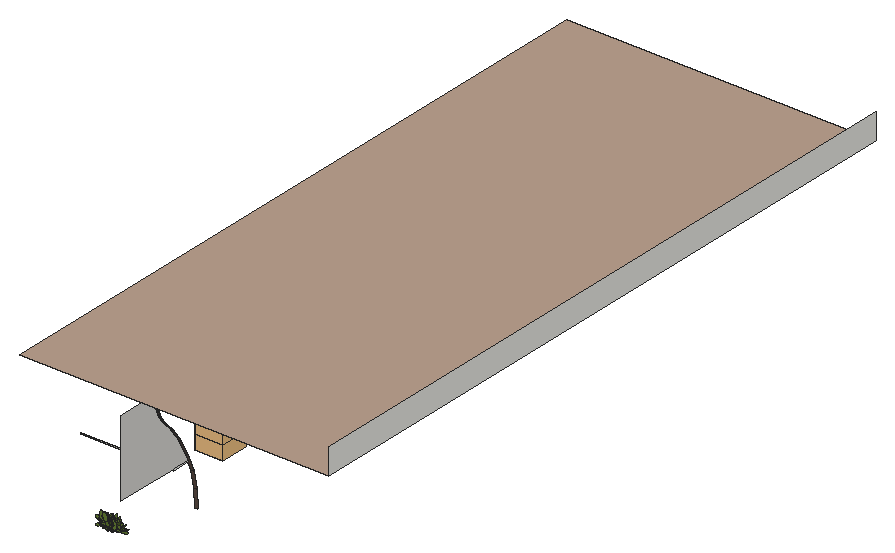
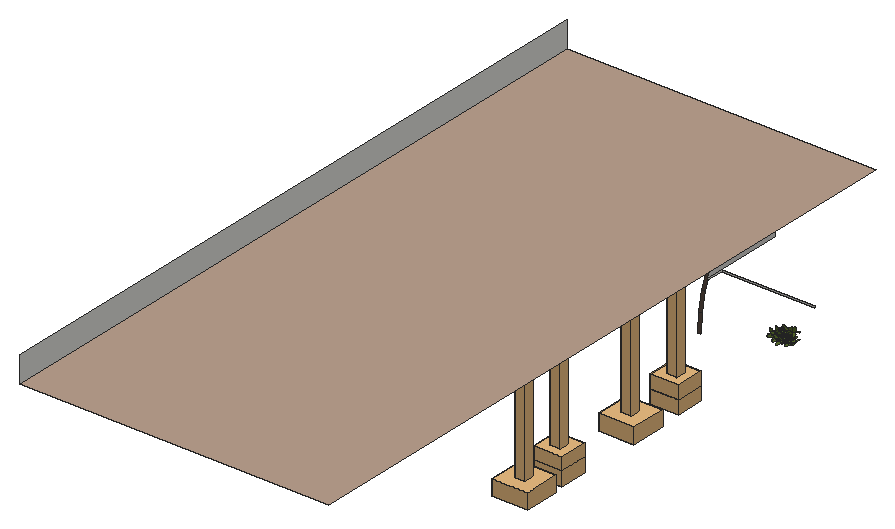
# SketchUp Ruby script. Lengths in inches.
U = 1.inch
M = Sketchup.active_model
def pt(a) = Geom::Point3d.new(a.map { |v| v * U })
def face(e, loops, mat)
  f = e.add_face(loops[0].map { |a| pt(a) })
  loops[1..].each { |l| e.add_face(l.map { |a| pt(a) }).erase! }
  f.material = f.back_material = mat if mat
  f
end
# faces: each face lists its corners as indices into pts; further lists are holes
def faces(e, pts, list, mat = nil) = list.each { |f| face(e, (f[0].is_a?(Array) ? f : [f]).map { |l| l.map { |i| pts[i] } }, mat) }
# xy, xz, yz: faces in a plane at the given z, y or x. An outline is a flat list of corners, or four numbers for a rectangle; further outlines are holes
def ring(l) = l.size == 4 ? [[l[0], l[1]], [l[2], l[1]], [l[2], l[3]], [l[0], l[3]]] : l.each_slice(2).to_a
def flat(e, list, mat, &to3) = list.each { |f| face(e, (f[0].is_a?(Array) ? f : [f]).map { |l| ring(l).map { |u, v| to3.(u, v) } }, mat) }
def xy(e, z, list, mat = nil) = flat(e, list, mat) { |x, y| [x, y, z] }
def xz(e, y, list, mat = nil) = flat(e, list, mat) { |x, z| [x, y, z] }
def yz(e, x, list, mat = nil) = flat(e, list, mat) { |y, z| [x, y, z] }
def lines(e, pts, list) = list.each { |a, b| e.add_line(pt(pts[a]), pt(pts[b])) }
# prism: a flat outline (further loops are holes) pulled along v
def prism(e, loops, v, mat = nil)
  f = face(e, loops, mat); d = Geom::Vector3d.new(v.map { |x| x * U })
  f.pushpull(f.normal.samedirection?(d) ? d.length : -d.length)
end
def box(e, o, s, mat = nil) = prism(e, [[o, [o[0] + s[0], o[1], o[2]], [o[0] + s[0], o[1] + s[1], o[2]], [o[0], o[1] + s[1], o[2]]]], [0, 0, s[2]], mat)
def at(x, y, z, deg = 0) = Geom::Transformation.translation(pt([x, y, z])) * Geom::Transformation.rotation(ORIGIN, Z_AXIS, deg.degrees)
def axes(o, x, y, z) = Geom::Transformation.new([*x, 0, *y, 0, *z, 0, *pt(o).to_a, 1])
def part(name) = M.definitions.add(name)
# library, detail: a bought-in or finely detailed component or shape, given as its bounding box
def library(name, o, s) = part(name).tap { |d| box(d.entities, o, s) }
def detail(e, o, s) = box(e.add_group.entities, o, s)
def put(e, d, t, mat = nil) = e.add_instance(d, t).tap { |i| i.material = mat if mat }
def group(e, t, mat = nil) = e.add_group.tap { |g| g.transformation = t; g.material = mat if mat }.entities
root = M.entities
M.materials.add("2").color = [91, 76, 69]
M.materials.add("[0008_LavenderBlush]").color = [212, 210, 207]
M.materials.add("[Asphalt_New]").color = [85, 106, 44]
M.materials.add("[Color A01]4").color = [188, 161, 143]
M.materials.add("white").color = [255, 255, 255]
c1 = part("Component\#59")
xy(c1.entities,0,[[5.79,0,4.75,0.06,3.73,0.22,2.73,0.5,1.77,0.88,0.86,1.37,0,1.95,0.83,2.59,1.74,3.13,2.7,3.56,3.7,3.87,4.74,4.05,5.79,4.12,6.84,4.05,7.87,3.87,8.88,3.56,9.84,3.13,10.74,2.59,11.57,1.95,10.72,1.37,9.8,0.88,8.84,0.5,7.84,0.22,6.82,0.06]],"[Asphalt_New]")
c2 = part("Leaf cluster")
put(c2.entities,c1,axes([10.37,9.23,1.73],[-0.67725,-0.67301,0.29729],[0.61625,-0.73963,-0.27052],[0.40195,0,0.91566]),"[Asphalt_New]")
put(c2.entities,c1,at(0,5.84,1.2),"[Asphalt_New]")
put(c2.entities,c1,axes([11.625,9.72,1.52],[-0.61694,-0.11161,0.77906],[-0.02647,-0.98639,-0.16227],[0.78657,-0.12073,0.60559]),"[Asphalt_New]")
put(c2.entities,c1,axes([13.35,8.05,1.98],[-0.1211,0.99122,-0.05316],[-0.90762,-0.13226,-0.39842],[-0.40195,0,0.91566]),"[Asphalt_New]")
c3 = library("Pendant light \#1",[-0.17,-0.17,-2.13],[2.36,2.36,31.14])
c4 = library("Group\#191",[0,0,0],[4.97,5,2.25])
c5 = library("Pendant light",[-0.17,-0.17,-2.23],[2.36,2.36,33.73])
c6 = library("Group\#195",[0,0,0],[6.25,6.23,2.75])
xy(root,126,[[125.375,9,197.1875,167.625]],"[Color A01]4")
xz(root,24.3,[[127.1875,103.38,148.875,103.78]],"[0008_LavenderBlush]")
yz(root,148.875,[[24.3,103.38,24.3,103.78,28.3,103.78,28.45,103.38]])
yz(root,148.875,[[9,103.78,9,121.625,18.35,121.625,18.35,122.4375,18.37,121.69,18.43,120.95,18.53,120.22,18.6875,119.49,18.89,118.78,19.14,118.08,19.4375,117.39,19.77,116.73,20.16,116.09,20.58,115.48,21.04,114.9,21.54,114.35,23.03,112.8,25.57,109.32,27.63,105.54,28.3,103.78]],"[0008_LavenderBlush]")
yz(root,197.1875,[[9,126,167.625,132]])
p = [[148.875,30.14,97.33],[149.5625,30.14,97.33],[149.5625,30.54,93.04],[148.875,30.54,93.04],[148.875,29.16,101.52],[149.5625,29.16,101.52],
  [148.875,27.63,105.54],[149.5625,27.63,105.54],[148.875,28.45,103.38],[148.875,28.3,103.78],[148.875,25.57,109.32],[149.5625,25.57,109.32],
  [148.875,23.03,112.8],[149.5625,23.03,112.8],[148.875,21.54,114.35],[149.5625,21.54,114.35],[148.875,21.04,114.9],[149.5625,21.04,114.9],
  [148.875,20.58,115.48],[149.5625,20.58,115.48],[148.875,20.16,116.09],[149.5625,20.16,116.09],[148.875,19.77,116.73],[149.5625,19.77,116.73],
  [148.875,19.4375,117.39],[149.5625,19.4375,117.39],[148.875,19.14,118.08],[149.5625,19.14,118.08],[148.875,18.89,118.78],[149.5625,18.89,118.78],
  [148.875,18.6875,119.49],[149.5625,18.6875,119.49],[148.875,18.53,120.22],[149.5625,18.53,120.22],[148.875,18.43,120.95],[149.5625,18.43,120.95],
  [148.875,18.37,121.69],[149.5625,18.37,121.69],[148.875,20.04,115.9],[149.5625,20.04,115.9]]
faces(root,p,[[0,1,2,3],[4,5,1,0],[6,7,5,4,8,9],[10,11,7,6],[12,13,11,10],[14,15,13,12],[14,16,17,15],[16,18,19,17],
  [18,20,21,19],[20,22,23,21],[22,24,25,23],[24,26,27,25],[26,28,29,27],[28,30,31,29],[30,32,33,31],[32,34,35,33],
  [34,36,37,35]],"2")
lines(root,p,[[38,39]])
detail(root,[134.31,48.47,92.11],[6.61,6.57,3.23])
detail(root,[134.31,82.33,92.11],[6.61,6.58,3.23])
put(root,c2,axes([138.4,18.32,90.67],[0.09591,-0.11801,0],[0.11801,0.09591,0],[0,0,0.17792]),"white")
put(root,c1,axes([136.48,18.12,90.71],[0.15184,-0.00221,-0.00946],[-0.00119,0.13948,-0.07089],[0.0083,0.06056,0.16292]),"[Asphalt_New]")
put(root,c2,axes([139,20.15,91.62],[-0.12334,-0.08896,0],[0.08896,-0.12334,0],[0,0,0.17792]),"white")
put(root,c2,axes([135.4,18.39,91.69],[0.09591,-0.11801,0],[0.11801,0.09591,0],[0,0,0.17792]),"white")
put(root,c1,axes([140.22,17.88,90.63],[-0.00707,0.09508,0.13861],[-0.14876,0.01968,-0.02887],[-0.03076,-0.11704,0.10775]),"[Asphalt_New]")
put(root,c2,axes([139.48,16.79,90.46],[0.12739,0.08305,0],[-0.08305,0.12739,0],[0,0,0.17792]),"white")
put(root,c2,axes([137.25,16.8125,90.89],[0.12739,0.08305,0],[-0.08305,0.12739,0],[0,0,0.17792]),"white")
put(root,c2,axes([139.18,20.1875,90.75],[-0.10525,-0.10976,0],[0.10976,-0.10525,0],[0,0,0.17792]),"white")
put(root,c2,axes([139.1,19.04,90.54],[-0.12303,0.08939,0],[-0.08939,-0.12303,0],[0,0,0.17792]),"white")
put(root,c1,axes([137.73,19.46,90.58],[-0.02064,-0.15066,0],[0.15066,-0.02064,0],[0,0,0.17792]),"[Asphalt_New]")
put(root,c1,axes([137.57,17.66,90.93],[0.01807,0.15078,-0.00946],[-0.13884,0.01339,-0.07089],[-0.05936,0.01458,0.16292]),"[Asphalt_New]")
put(root,c1,axes([140.16,18.08,90.67],[-0.09102,0.11312,0.0529],[-0.12166,-0.08144,-0.04813],[-0.00639,-0.06079,0.16292]),"[Asphalt_New]")
put(root,c1,axes([138.08,18.27,90.71],[0.15183,0.00256,-0.00946],[-0.00557,0.13937,-0.07089],[0.00639,0.06079,0.16292]),"[Asphalt_New]")
put(root,c1,axes([140.07,17.97,90.42],[-0.00408,0.09525,0.13861],[-0.14807,0.02435,-0.02887],[-0.03442,-0.11602,0.10775]),"[Asphalt_New]")
put(root,c1,axes([140.79,17.75,90.67],[0.10299,0.10235,0.0529],[-0.09371,0.11248,-0.04813],[-0.06112,0,0.16292]),"[Asphalt_New]")
put(root,c2,axes([141.9,19.1,90.54],[-0.12303,0.08939,0],[-0.08939,-0.12303,0],[0,0,0.17792]),"white")
put(root,c2,axes([137.49,16.9,90.67],[0.12994,0.079,0],[-0.079,0.12994,0],[0,0,0.17792]),"white")
put(root,c1,axes([140.16,18.92,90.89],[-0.15207,0,0],[0,-0.15207,0],[0,0,0.17792]),"[Asphalt_New]")
put(root,c2,axes([136.17,18.03,91.48],[0.1271,-0.08349,0],[0.08349,0.1271,0],[0,0,0.17792]),"white")
put(root,c1,axes([137.79,17.82,91.69],[0.10299,0.10235,0.0529],[-0.09371,0.11248,-0.04813],[-0.06112,0,0.16292]),"[Asphalt_New]")
put(root,c1,axes([137.83,18.0625,90.85],[-0.00408,0.09525,0.13861],[-0.14807,0.02435,-0.02887],[-0.03442,-0.11602,0.10775]),"[Asphalt_New]")
put(root,c1,axes([140.02,18.17,90.46],[-0.08742,0.11593,0.0529],[-0.12415,-0.07758,-0.04813],[-0.0083,-0.06056,0.16292]),"[Asphalt_New]")
put(root,c1,axes([139.58,18.13,90.63],[-0.00707,0.09508,0.13861],[-0.14876,0.01968,-0.02887],[-0.03076,-0.11704,0.10775]),"[Asphalt_New]")
put(root,c1,axes([138.39,18.33,90.94],[0.09382,0.01697,0.13861],[0.00402,0.15,-0.02887],[-0.11961,0.01836,0.10775]),"[Asphalt_New]")
put(root,c1,axes([138.96,17.85,90.93],[0.01807,0.15078,-0.00946],[-0.13884,0.01339,-0.07089],[-0.05936,0.01458,0.16292]),"[Asphalt_New]")
put(root,c1,axes([137.79,18.26,90.88],[-0.08742,0.11593,0.0529],[-0.12415,-0.07758,-0.04813],[-0.0083,-0.06056,0.16292]),"[Asphalt_New]")
put(root,c2,axes([138.18,20.46,90.54],[-0.10525,-0.10976,0],[0.10976,-0.10525,0],[0,0,0.17792]),"white")
put(root,c1,axes([139.81,19.7,90.58],[-0.0159,-0.15124,0],[0.15124,-0.0159,0],[0,0,0.17792]),"[Asphalt_New]")
put(root,c2,axes([138.97,17.11,90.67],[0.12739,0.08305,0],[-0.08305,0.12739,0],[0,0,0.17792]),"white")
put(root,c1,axes([139.52,18.33,90.67],[-0.09102,0.11312,0.0529],[-0.12166,-0.08144,-0.04813],[-0.00639,-0.06079,0.16292]),"[Asphalt_New]")
put(root,c2,axes([136.53,20.4,90.52],[-0.06975,-0.13513,0],[0.13513,-0.06975,0],[0,0,0.17792]),"white")
put(root,c1,axes([139.73,19.8,90.36],[-0.02064,-0.15066,0],[0.15066,-0.02064,0],[0,0,0.17792]),"[Asphalt_New]")
put(root,c1,axes([139.5625,18.31,90.63],[-0.00408,0.09525,0.13861],[-0.14807,0.02435,-0.02887],[-0.03442,-0.11602,0.10775]),"[Asphalt_New]")
put(root,c1,axes([136.98,18.1,90.7],[-0.0255,0.1497,-0.00946],[-0.13692,-0.02659,-0.07089],[-0.06106,-0.00288,0.16292]),"[Asphalt_New]")
put(root,c1,axes([139.61,19.24,90.89],[-0.15207,0,0],[0,-0.15207,0],[0,0,0.17792]),"[Asphalt_New]")
put(root,c1,axes([140.07,18.67,90.5],[0.15183,0.00256,-0.00946],[-0.00557,0.13937,-0.07089],[0.00639,0.06079,0.16292]),"[Asphalt_New]")
put(root,c1,axes([137.49,19.89,90.79],[-0.02064,-0.15066,0],[0.15066,-0.02064,0],[0,0,0.17792]),"[Asphalt_New]")
put(root,c1,axes([137.83,18.7,90.93],[0.15183,0.00256,-0.00946],[-0.00557,0.13937,-0.07089],[0.00639,0.06079,0.16292]),"[Asphalt_New]")
put(root,c1,axes([139.52,18.51,90.67],[-0.08742,0.11593,0.0529],[-0.12415,-0.07758,-0.04813],[-0.0083,-0.06056,0.16292]),"[Asphalt_New]")
put(root,c1,axes([137.96,18.125,90.71],[0.01807,0.15078,-0.00946],[-0.13884,0.01339,-0.07089],[-0.05936,0.01458,0.16292]),"[Asphalt_New]")
put(root,c2,axes([136.19,18.96,90.98],[0.09591,-0.11801,0],[0.11801,0.09591,0],[0,0,0.17792]),"white")
put(root,c1,axes([138.14,18.77,90.71],[0.15184,-0.00221,-0.00946],[-0.00119,0.13948,-0.07089],[0.0083,0.06056,0.16292]),"[Asphalt_New]")
put(root,c1,axes([139.17,19.95,90.58],[-0.0159,-0.15124,0],[0.15124,-0.0159,0],[0,0,0.17792]),"[Asphalt_New]")
put(root,c1,axes([142.5,19.36,90.36],[-0.15207,0,0],[0,-0.15207,0],[0,0,0.17792]),"[Asphalt_New]")
put(root,c1,axes([137.84,18.65,90.94],[0.09382,0.01697,0.13861],[0.00402,0.15,-0.02887],[-0.11961,0.01836,0.10775]),"[Asphalt_New]")
put(root,c1,axes([138.36,18.5,90.63],[-0.00707,0.09508,0.13861],[-0.14876,0.01968,-0.02887],[-0.03076,-0.11704,0.10775]),"[Asphalt_New]")
put(root,c1,axes([140.73,18.78,90.42],[0.09382,0.01697,0.13861],[0.00402,0.15,-0.02887],[-0.11961,0.01836,0.10775]),"[Asphalt_New]")
put(root,c1,axes([138.3125,18.7,90.67],[-0.09102,0.11312,0.0529],[-0.12166,-0.08144,-0.04813],[-0.00639,-0.06079,0.16292]),"[Asphalt_New]")
put(root,c1,axes([138.58,18.4,90.98],[0.10299,0.10235,0.0529],[-0.09371,0.11248,-0.04813],[-0.06112,0,0.16292]),"[Asphalt_New]")
put(root,c1,axes([139.22,20.14,90.58],[-0.02064,-0.15066,0],[0.15066,-0.02064,0],[0,0,0.17792]),"[Asphalt_New]")
put(root,c2,axes([140.73,19.74,90.54],[-0.12303,0.08939,0],[-0.08939,-0.12303,0],[0,0,0.17792]),"white")
put(root,c1,axes([136.76,18.9375,90.71],[0.15183,0.00256,-0.00946],[-0.00557,0.13937,-0.07089],[0.00639,0.06079,0.16292]),"[Asphalt_New]")
put(root,c1,axes([136.42,20.17,90.58],[-0.02064,-0.15066,0],[0.15066,-0.02064,0],[0,0,0.17792]),"[Asphalt_New]")
put(root,c1,axes([139.55,19,90.71],[0.15183,0.00256,-0.00946],[-0.00557,0.13937,-0.07089],[0.00639,0.06079,0.16292]),"[Asphalt_New]")
put(root,c2,axes([135.65,19.29,90.98],[0.09591,-0.11801,0],[0.11801,0.09591,0],[0,0,0.17792]),"white")
put(root,c1,axes([137.96,20.32,90.58],[-0.0159,-0.15124,0],[0.15124,-0.0159,0],[0,0,0.17792]),"[Asphalt_New]")
put(root,c2,axes([137.81,17.76,90.67],[0.12739,0.08305,0],[-0.08305,0.12739,0],[0,0,0.17792]),"white")
put(root,c2,axes([138.53,19.41,90.46],[0.09591,-0.11801,0],[0.11801,0.09591,0],[0,0,0.17792]),"white")
put(root,c1,axes([140.35,18.91,90.42],[-0.00707,0.09508,0.13861],[-0.14876,0.01968,-0.02887],[-0.03076,-0.11704,0.10775]),"[Asphalt_New]")
put(root,c1,axes([138.11,18.93,90.85],[-0.00707,0.09508,0.13861],[-0.14876,0.01968,-0.02887],[-0.03076,-0.11704,0.10775]),"[Asphalt_New]")
put(root,c1,axes([138.03,18.72,90.98],[0.10299,0.10235,0.0529],[-0.09371,0.11248,-0.04813],[-0.06112,0,0.16292]),"[Asphalt_New]")
put(root,c1,axes([138.42,18.99,90.63],[-0.00408,0.09525,0.13861],[-0.14807,0.02435,-0.02887],[-0.03442,-0.11602,0.10775]),"[Asphalt_New]")
put(root,c1,axes([140.3,19.11,90.46],[-0.09102,0.11312,0.0529],[-0.12166,-0.08144,-0.04813],[-0.00639,-0.06079,0.16292]),"[Asphalt_New]")
put(root,c1,axes([138.06,19.125,90.88],[-0.09102,0.11312,0.0529],[-0.12166,-0.08144,-0.04813],[-0.00639,-0.06079,0.16292]),"[Asphalt_New]")
put(root,c1,axes([138.375,19.19,90.67],[-0.08742,0.11593,0.0529],[-0.12415,-0.07758,-0.04813],[-0.0083,-0.06056,0.16292]),"[Asphalt_New]")
put(root,c1,axes([137.03,19.17,90.63],[-0.00707,0.09508,0.13861],[-0.14876,0.01968,-0.02887],[-0.03076,-0.11704,0.10775]),"[Asphalt_New]")
put(root,c1,axes([139.95,20.73,90.36],[-0.0159,-0.15124,0],[0.15124,-0.0159,0],[0,0,0.17792]),"[Asphalt_New]")
put(root,c1,axes([139.83,19.23,90.63],[-0.00707,0.09508,0.13861],[-0.14876,0.01968,-0.02887],[-0.03076,-0.11704,0.10775]),"[Asphalt_New]")
put(root,c1,axes([137.71,20.75,90.79],[-0.0159,-0.15124,0],[0.15124,-0.0159,0],[0,0,0.17792]),"[Asphalt_New]")
put(root,c1,axes([138.08,20.82,90.58],[-0.02064,-0.15066,0],[0.15066,-0.02064,0],[0,0,0.17792]),"[Asphalt_New]")
put(root,c1,axes([139.78,19.43,90.67],[-0.09102,0.11312,0.0529],[-0.12166,-0.08144,-0.04813],[-0.00639,-0.06079,0.16292]),"[Asphalt_New]")
put(root,c1,axes([138.39,19.64,90.71],[0.15183,0.00256,-0.00946],[-0.00557,0.13937,-0.07089],[0.00639,0.06079,0.16292]),"[Asphalt_New]")
put(root,c1,axes([136.63,20.99,90.58],[-0.0159,-0.15124,0],[0.15124,-0.0159,0],[0,0,0.17792]),"[Asphalt_New]")
put(root,c1,axes([139.43,21.05,90.58],[-0.0159,-0.15124,0],[0.15124,-0.0159,0],[0,0,0.17792]),"[Asphalt_New]")
put(root,c1,axes([138.67,19.875,90.63],[-0.00707,0.09508,0.13861],[-0.14876,0.01968,-0.02887],[-0.03076,-0.11704,0.10775]),"[Asphalt_New]")
put(root,c1,axes([138.62,20.07,90.67],[-0.09102,0.11312,0.0529],[-0.12166,-0.08144,-0.04813],[-0.00639,-0.06079,0.16292]),"[Asphalt_New]")
put(root,c1,axes([138.27,21.69,90.58],[-0.0159,-0.15124,0],[0.15124,-0.0159,0],[0,0,0.17792]),"[Asphalt_New]")
put(root,c3,at(136.63,52.72,94.67,-90))
put(root,c4,axes([134.31,55.04,95.34],[0,-1.3225,0],[1.3225,0,0],[0,0,1.3225]))
put(root,c5,at(137.31,65.14,91.9375,-90))
put(root,c6,axes([134.13,68.27,91.84],[0,-1.3225,0],[1.3225,0,0],[0,0,1.3225]))
put(root,c3,at(136.63,86.59,94.67,-90))
put(root,c4,axes([134.31,88.91,95.34],[0,-1.3225,0],[1.3225,0,0],[0,0,1.3225]))
put(root,c5,at(137.31,96.05,91.9375,-90))
put(root,c6,axes([134.13,99.18,91.84],[0,-1.3225,0],[1.3225,0,0],[0,0,1.3225]))
